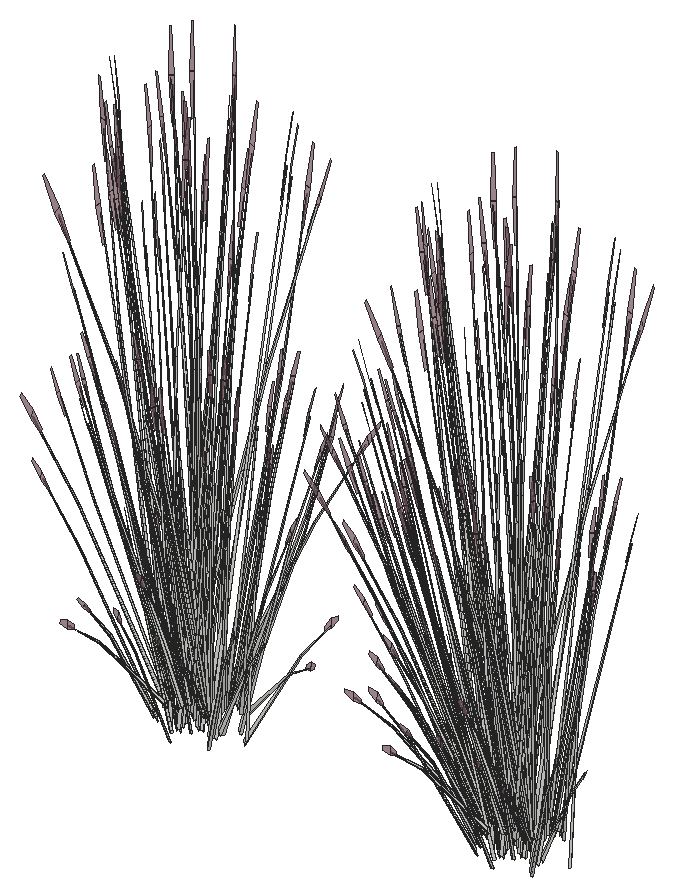
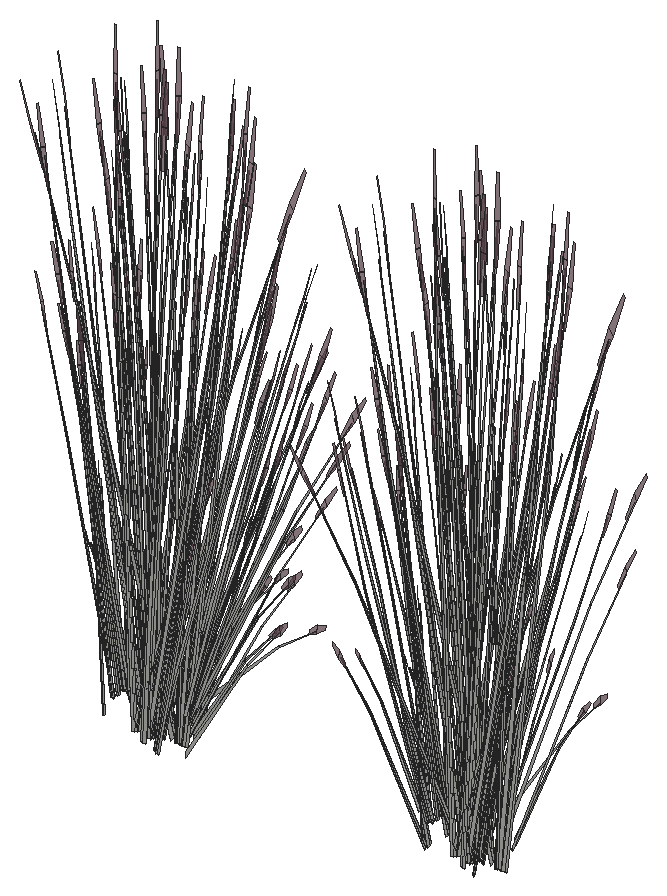
# SketchUp Ruby script. Lengths in inches.
U = 1.inch
M = Sketchup.active_model
def pt(a) = Geom::Point3d.new(a.map { |v| v * U })
def face(e, loops, mat)
  f = e.add_face(loops[0].map { |a| pt(a) })
  loops[1..].each { |l| e.add_face(l.map { |a| pt(a) }).erase! }
  f.material = f.back_material = mat if mat
  f
end
# faces: each face lists its corners as indices into pts; further lists are holes
def faces(e, pts, list, mat = nil) = list.each { |f| face(e, (f[0].is_a?(Array) ? f : [f]).map { |l| l.map { |i| pts[i] } }, mat) }
# xy, xz, yz: faces in a plane at the given z, y or x. An outline is a flat list of corners, or four numbers for a rectangle; further outlines are holes
def ring(l) = l.size == 4 ? [[l[0], l[1]], [l[2], l[1]], [l[2], l[3]], [l[0], l[3]]] : l.each_slice(2).to_a
def flat(e, list, mat, &to3) = list.each { |f| face(e, (f[0].is_a?(Array) ? f : [f]).map { |l| ring(l).map { |u, v| to3.(u, v) } }, mat) }
def xy(e, z, list, mat = nil) = flat(e, list, mat) { |x, y| [x, y, z] }
def xz(e, y, list, mat = nil) = flat(e, list, mat) { |x, z| [x, y, z] }
def yz(e, x, list, mat = nil) = flat(e, list, mat) { |y, z| [x, y, z] }
def lines(e, pts, list) = list.each { |a, b| e.add_line(pt(pts[a]), pt(pts[b])) }
# prism: a flat outline (further loops are holes) pulled along v
def prism(e, loops, v, mat = nil)
  f = face(e, loops, mat); d = Geom::Vector3d.new(v.map { |x| x * U })
  f.pushpull(f.normal.samedirection?(d) ? d.length : -d.length)
end
def box(e, o, s, mat = nil) = prism(e, [[o, [o[0] + s[0], o[1], o[2]], [o[0] + s[0], o[1] + s[1], o[2]], [o[0], o[1] + s[1], o[2]]]], [0, 0, s[2]], mat)
def at(x, y, z, deg = 0) = Geom::Transformation.translation(pt([x, y, z])) * Geom::Transformation.rotation(ORIGIN, Z_AXIS, deg.degrees)
def axes(o, x, y, z) = Geom::Transformation.new([*x, 0, *y, 0, *z, 0, *pt(o).to_a, 1])
def part(name) = M.definitions.add(name)
# library, detail: a bought-in or finely detailed component or shape, given as its bounding box
def library(name, o, s) = part(name).tap { |d| box(d.entities, o, s) }
def detail(e, o, s) = box(e.add_group.entities, o, s)
def put(e, d, t, mat = nil) = e.add_instance(d, t).tap { |i| i.material = mat if mat }
def group(e, t, mat = nil) = e.add_group.tap { |g| g.transformation = t; g.material = mat if mat }.entities
root = M.entities
M.materials.add("LightPink_Translucent").color = [144, 107, 117]
M.materials["LightPink_Translucent"].alpha = 0.75
c1 = part("blade")
p = [[2.15,0.21,22],[0,0.17,0],[0.09,0.45,0],[2.18,0.31,22],[2.29,0.31,22],[0.38,0.45,0],
  [2.48,0.24,33],[2.49,0.24,33],[2.48,0.22,33]]
faces(c1.entities,p,[[0,1,2,3],[4,5,2,3],[6,3,4,7],[8,0,3,6]])
c2 = part("seeds")
p = [[0.3,-0.1,1.38],[-0.01,-0.03,1.59],[-0.01,-0.03,0.03],[0.14,-0.07,-0.07],[0.29,-0.03,3],[0.15,0.01,3.11]]
faces(c2.entities,p,[[0,1,2,3],[1,0,4,5]],"LightPink_Translucent")
c3 = part("blade with seeds")
put(c3.entities,c1,at(0,0,0))
put(c3.entities,c2,axes([2.4,0.25,30.99],[1.5799,-0.05474,1.17369],[-0.12525,1.92788,0.29478],[-0.07173,-0.02425,1.56792]))
put(root,c3,axes([282.12,10.6,-2.125],[0.17368,0.19618,1.71376],[-0.80256,0.16516,0.13857],[-0.18139,-0.30799,0.73262]))
put(root,c3,axes([314.91,10.6,-2.125],[0.17368,0.19618,1.71376],[-0.80256,0.16516,0.13857],[-0.18139,-0.30799,0.73262]))
put(root,c3,axes([283.44,9.3,-1.28],[-0.11621,-0.08567,1.74944],[-0.77555,0.05431,-0.27667],[-0.12378,-0.20491,0.14031]))
put(root,c3,axes([316.24,9.3,-1.28],[-0.11621,-0.08567,1.74944],[-0.77555,0.05431,-0.27667],[-0.12378,-0.20491,0.14031]))
put(root,c3,axes([285.24,10.3125,-3.41],[-0.21597,0.12368,1.43002],[-0.64681,-0.21647,-0.30754],[0.1199,-0.26922,0.61141]))
put(root,c3,axes([318.03,10.3125,-3.41],[-0.21597,0.12368,1.43002],[-0.64681,-0.21647,-0.30754],[0.1199,-0.26922,0.61141]))
put(root,c3,axes([284.26,10.74,-1.02],[-0.36264,-0.49684,-0.71045],[0.74649,-0.27689,0.08574],[-0.0848,-0.24006,1.00501]))
put(root,c3,axes([317.05,10.74,-1.02],[-0.36264,-0.49684,-0.71045],[0.74649,-0.27689,0.08574],[-0.0848,-0.24006,1.00501]))
put(root,c3,axes([281.9,10.08,-3.41],[-0.04601,0.19989,1.43002],[-0.67263,0.16733,-0.30754],[-0.15723,-0.25836,0.61141]))
put(root,c3,axes([314.69,10.08,-3.41],[-0.04601,0.19989,1.43002],[-0.67263,0.16733,-0.30754],[-0.15723,-0.25836,0.61141]))
put(root,c3,axes([283.63,9.64,-4.51],[-0.12744,0.02202,1.76342],[-0.70477,-0.24781,-0.26939],[0.01183,-0.2067,0.30037]))
put(root,c3,axes([316.42,9.64,-4.51],[-0.12744,0.02202,1.76342],[-0.70477,-0.24781,-0.26939],[0.01183,-0.2067,0.30037]))
put(root,c3,axes([285.77,11.23,-1.02],[0.01977,-0.56521,-0.71045],[0.83252,0.03796,0.08574],[0.08786,-0.23945,1.00501]))
put(root,c3,axes([318.56,11.23,-1.02],[0.01977,-0.56521,-0.71045],[0.83252,0.03796,0.08574],[0.08786,-0.23945,1.00501]))
put(root,c3,axes([286.93,10.35,-1.28],[-0.00733,-0.12161,1.74944],[-0.61946,-0.35147,-0.27667],[0.09577,-0.21306,0.14031]))
put(root,c3,axes([319.72,10.35,-1.28],[-0.00733,-0.12161,1.74944],[-0.61946,-0.35147,-0.27667],[0.09577,-0.21306,0.14031]))
put(root,c3,axes([284.32,10.32,-1.47],[0.22906,-0.4699,-0.35414],[0.66828,0.13705,0.4572],[-0.06128,-0.18919,0.87481]))
put(root,c3,axes([317.12,10.32,-1.47],[0.22906,-0.4699,-0.35414],[0.66828,0.13705,0.4572],[-0.06128,-0.18919,0.87481]))
put(root,c3,axes([284.83,10.94,-2.125],[-0.14147,0.21002,1.71376],[-0.59349,-0.43464,0.13857],[0.26773,-0.27089,0.73262]))
put(root,c3,axes([317.62,10.94,-2.125],[-0.14147,0.21002,1.71376],[-0.59349,-0.43464,0.13857],[0.26773,-0.27089,0.73262]))
put(root,c3,axes([286.76,9.91,-1.29],[-0.07716,0.04667,1.77383],[-0.75601,-0.15746,-0.16761],[-0.02737,-0.20368,0.31391]))
put(root,c3,axes([319.55,9.91,-1.29],[-0.07716,0.04667,1.77383],[-0.75601,-0.15746,-0.16761],[-0.02737,-0.20368,0.31391]))
put(root,c3,axes([283.98,10.64,-1.32],[-0.7469,-0.15318,-0.51099],[0.25601,-0.52518,-0.3958],[-0.06849,-0.21144,0.97773]))
put(root,c3,axes([316.78,10.64,-1.32],[-0.7469,-0.15318,-0.51099],[0.25601,-0.52518,-0.3958],[-0.06849,-0.21144,0.97773]))
put(root,c3,axes([284.45,9.33,-3.23],[0.09747,0.35631,1.1486],[-0.54071,-0.19735,0.84392],[0.05818,-0.18244,0.25299]))
put(root,c3,axes([317.24,9.33,-3.23],[0.09747,0.35631,1.1486],[-0.54071,-0.19735,0.84392],[0.05818,-0.18244,0.25299]))
put(root,c3,axes([285.6,11.04,-1.32],[-0.54391,-0.41056,-0.51099],[0.57458,-0.35956,-0.3958],[0.08276,-0.2086,0.97773]))
put(root,c3,axes([318.39,11.04,-1.32],[-0.54391,-0.41056,-0.51099],[0.57458,-0.35956,-0.3958],[0.08276,-0.2086,0.97773]))
put(root,c3,axes([315.44,9.02,-1.29],[-0.01417,0.07324,1.77383],[-0.6991,0.2658,-0.16761],[-0.20573,-0.13587,0.31391]))
put(root,c3,axes([282.49,10.31,-0.91],[0.84639,-0.15705,0.53763],[0.14689,0.61608,0.4433],[-0.19906,-0.18157,1.11249]))
put(root,c3,axes([315.29,10.31,-0.91],[0.84639,-0.15705,0.53763],[0.14689,0.61608,0.4433],[-0.19906,-0.18157,1.11249]))
put(root,c3,axes([284.41,10.43,-1.27],[0.74868,0.15974,0.48003],[-0.25601,0.52518,0.3958],[-0.04499,-0.20653,0.9933]))
put(root,c3,axes([317.2,10.43,-1.27],[0.74868,0.15974,0.48003],[-0.25601,0.52518,0.3958],[-0.04499,-0.20653,0.9933]))
put(root,c3,axes([284.62,10.62,-0.97],[-0.74352,0.28449,-0.1216],[-0.36538,-0.50492,-0.67495],[-0.0981,-0.21277,1.02557]))
put(root,c3,axes([317.42,10.62,-0.97],[-0.74352,0.28449,-0.1216],[-0.36538,-0.50492,-0.67495],[-0.0981,-0.21277,1.02557]))
put(root,c3,axes([286.17,11.26,-0.97],[-0.83505,-0.03027,-0.1216],[0.02282,-0.57322,-0.67495],[0.05801,-0.22077,1.02557]))
put(root,c3,axes([318.96,11.26,-0.97],[-0.83505,-0.03027,-0.1216],[0.02282,-0.57322,-0.67495],[0.05801,-0.22077,1.02557]))
put(root,c3,axes([286.11,10.89,-1.47],[0.5141,-0.32171,-0.35414],[0.48666,0.36734,0.4572],[0.07405,-0.18664,0.87481]))
put(root,c3,axes([318.9,10.89,-1.47],[0.5141,-0.32171,-0.35414],[0.48666,0.36734,0.4572],[0.07405,-0.18664,0.87481]))
put(root,c3,axes([281.67,9.76,-3.23],[0.39634,0.21267,1.1486],[-0.57721,0.12784,0.84392],[-0.1235,-0.16344,0.25299]))
put(root,c3,axes([314.46,9.76,-3.23],[0.39634,0.21267,1.1486],[-0.57721,0.12784,0.84392],[-0.1235,-0.16344,0.25299]))
put(root,c3,axes([284.61,10.39,-1.27],[0.55987,-0.20767,0.0643],[0.27403,0.37869,0.50621],[-0.05407,-0.16693,0.77189]))
put(root,c3,axes([317.4,10.39,-1.27],[0.55987,-0.20767,0.0643],[0.27403,0.37869,0.50621],[-0.05407,-0.16693,0.77189]))
put(root,c3,axes([315.42,10.88,-1.02],[-0.64788,-0.29534,-0.71045],[0.46044,-0.51755,0.08574],[-0.23473,-0.17635,1.00501]))
put(root,c3,axes([282.4,10.49,-1.47],[-0.11735,-0.49217,-0.35414],[0.67083,-0.12996,0.4572],[-0.18018,-0.14104,0.87481]))
put(root,c3,axes([315.19,10.49,-1.47],[-0.11735,-0.49217,-0.35414],[0.67083,-0.12996,0.4572],[-0.18018,-0.14104,0.87481]))
put(root,c3,axes([282.6875,10.45,-1.27],[0.34533,-0.38816,0.0643],[0.49176,0.22599,0.50621],[-0.15898,-0.12445,0.77189]))
put(root,c3,axes([315.48,10.45,-1.27],[0.34533,-0.38816,0.0643],[0.49176,0.22599,0.50621],[-0.15898,-0.12445,0.77189]))
put(root,c3,axes([314.15,10.4,-4.51],[-0.0736,0.08049,1.76342],[-0.74378,0.17355,-0.26939],[-0.17968,-0.15788,0.30037]))
put(root,c3,axes([282.58,12.61,-3.9],[-0.31203,-0.62659,-0.69835],[0.89884,-0.22566,-0.18329],[-0.03449,-0.21218,1.54149]))
put(root,c3,axes([315.37,12.61,-3.9],[-0.31203,-0.62659,-0.69835],[0.89884,-0.22566,-0.18329],[-0.03449,-0.21218,1.54149]))
put(root,c3,axes([313.75,11.21,-2.125],[0.28223,0.10528,1.71376],[-0.58406,0.44165,0.13857],[-0.36402,-0.19924,0.73262]))
put(root,c3,axes([286.75,10.69,-4.51],[-0.11372,-0.04814,1.76342],[-0.29211,-0.53779,-0.26939],[0.19706,-0.14594,0.30037]))
put(root,c3,axes([319.54,10.69,-4.51],[-0.11372,-0.04814,1.76342],[-0.29211,-0.53779,-0.26939],[0.19706,-0.14594,0.30037]))
put(root,c3,axes([284.4,10.82,-0.95],[-0.22906,0.4699,0.35414],[-0.66828,-0.13705,-0.4572],[-0.06128,-0.18919,0.87481]))
put(root,c3,axes([317.19,10.82,-0.95],[-0.22906,0.4699,0.35414],[-0.66828,-0.13705,-0.4572],[-0.06128,-0.18919,0.87481]))
put(root,c3,axes([315.11,10.9,-1.32],[-0.74975,0.14525,-0.51099],[-0.13115,-0.55007,-0.3958],[-0.20138,-0.15763,0.97773]))
put(root,c3,axes([286.11,11.01,-1.27],[0.54105,0.41691,0.48003],[-0.57458,0.35956,0.3958],[0.0998,-0.1956,0.9933]))
put(root,c3,axes([318.9,11.01,-1.27],[0.54105,0.41691,0.48003],[-0.57458,0.35956,0.3958],[0.0998,-0.1956,0.9933]))
put(root,c3,axes([315.64,10.41,-0.57],[-0.50709,0.58578,-0.13619],[-0.73436,-0.33748,-0.75594],[-0.25527,-0.1655,1.14864]))
put(root,c3,axes([286.31,11.05,-1.27],[0.62439,0.02847,0.0643],[-0.01712,0.42991,0.50621],[0.06534,-0.16468,0.77189]))
put(root,c3,axes([319.1,11.05,-1.27],[0.62439,0.02847,0.0643],[-0.01712,0.42991,0.50621],[0.06534,-0.16468,0.77189]))
put(root,c3,axes([285.84,11.35,-0.95],[-0.5141,0.32171,0.35414],[-0.48666,-0.36734,-0.4572],[0.07405,-0.18664,0.87481]))
put(root,c3,axes([318.63,11.35,-0.95],[-0.5141,0.32171,0.35414],[-0.48666,-0.36734,-0.4572],[0.07405,-0.18664,0.87481]))
put(root,c3,axes([286.75,12.21,-1.02],[0.39688,-0.48213,-0.71045],[0.69548,0.34264,0.08574],[0.23697,-0.17468,1.00501]))
put(root,c3,axes([319.54,12.21,-1.02],[0.39688,-0.48213,-0.71045],[0.69548,0.34264,0.08574],[0.23697,-0.17468,1.00501]))
put(root,c3,axes([282.46,10.81,-3.625],[-0.47504,-0.61229,0],[0.79476,-0.34146,-0.51607],[0.18101,-0.07777,1.63711]))
put(root,c3,axes([315.25,10.81,-3.625],[-0.47504,-0.61229,0],[0.79476,-0.34146,-0.51607],[0.18101,-0.07777,1.63711]))
put(root,c3,axes([286.73,11.99,-1.32],[-0.19519,-0.55794,-0.51099],[0.73919,-0.0976,-0.3958],[0.21183,-0.14986,0.97773]))
put(root,c3,axes([319.52,11.99,-1.32],[-0.19519,-0.55794,-0.51099],[0.73919,-0.0976,-0.3958],[0.21183,-0.14986,0.97773]))
put(root,c3,axes([283.5,10.07,-3.87],[-0.52505,0.35054,-0.03893],[-0.48109,-0.38392,-0.17649],[-0.03387,-0.10878,0.58215]))
put(root,c3,axes([316.29,10.07,-3.87],[-0.52505,0.35054,-0.03893],[-0.48109,-0.38392,-0.17649],[-0.03387,-0.10878,0.58215]))
put(root,c3,axes([313.69,10.24,-1.28],[-0.16348,-0.00431,1.74944],[-0.52047,0.43131,-0.27667],[-0.2777,-0.08813,0.14031]))
put(root,c3,axes([287.08,12.39,-0.97],[-0.70283,-0.33692,-0.1216],[0.40491,-0.48793,-0.67495],[0.19857,-0.16961,1.02557]))
put(root,c3,axes([319.87,12.39,-0.97],[-0.70283,-0.33692,-0.1216],[0.40491,-0.48793,-0.67495],[0.19857,-0.16961,1.02557]))
put(root,c3,axes([284.17,14.22,-2.67],[0.65659,0.2464,1.51261],[-0.64324,0.53082,0.59816],[-0.28812,-0.31461,1.26806]))
put(root,c3,axes([316.97,14.22,-2.67],[0.65659,0.2464,1.51261],[-0.64324,0.53082,0.59816],[-0.28812,-0.31461,1.26806]))
put(root,c3,axes([282.79,10.89,-0.95],[0.11735,0.49217,0.35414],[-0.67083,0.12996,-0.4572],[-0.18018,-0.14104,0.87481]))
put(root,c3,axes([315.59,10.89,-0.95],[0.11735,0.49217,0.35414],[-0.67083,0.12996,-0.4572],[-0.18018,-0.14104,0.87481]))
put(root,c3,axes([280.74,12.52,-3.98],[0,-0.61104,-0.49651],[0.85008,0,0],[0,-0.13917,1.57504]))
put(root,c3,axes([313.53,12.52,-3.98],[0,-0.61104,-0.49651],[0.85008,0,0],[0,-0.13917,1.57504]))
put(root,c3,axes([283.1,10.71,-3.98],[0.7111,-0.30552,-0.49651],[0.42504,0.54784,0],[0.16196,-0.06958,1.57504]))
put(root,c3,axes([315.9,10.71,-3.98],[0.7111,-0.30552,-0.49651],[0.42504,0.54784,0],[0.16196,-0.06958,1.57504]))
put(root,c3,axes([287.32,11.77,-3.41],[-0.27143,-0.0181,1.43002],[-0.27808,-0.48551,-0.30754],[0.33346,-0.13735,0.61141]))
put(root,c3,axes([313.57,11.21,-0.91],[0.62747,-0.45094,0.53763],[0.54116,0.47889,0.4433],[-0.29439,-0.08318,1.11249]))
put(root,c3,axes([288.81,12.24,-1.29],[-0.09924,-0.00464,1.77383],[-0.4121,-0.49725,-0.16761],[0.1655,-0.1635,0.31391]))
put(root,c3,axes([321.6,12.24,-1.29],[-0.09924,-0.00464,1.77383],[-0.4121,-0.49725,-0.16761],[0.1655,-0.1635,0.31391]))
put(root,c3,axes([283.94,11.97,-3.94],[0.51177,-0.45928,-0.62353],[0.63575,0.41646,-0.16365],[0.20507,-0.11457,1.37633]))
put(root,c3,axes([316.74,11.97,-3.94],[0.51177,-0.45928,-0.62353],[0.63575,0.41646,-0.16365],[0.20507,-0.11457,1.37633]))
put(root,c3,axes([287.63,10.875,-3.23],[-0.25308,0.31105,1.1486],[-0.21753,-0.4179,0.84392],[0.20902,-0.10472,0.25299]))
put(root,c3,axes([320.43,10.875,-3.23],[-0.25308,0.31105,1.1486],[-0.21753,-0.4179,0.84392],[0.20902,-0.10472,0.25299]))
put(root,c3,axes([287.27,12.04,-1.47],[0.66138,-0.08733,-0.35414],[0.17464,0.49921,0.4572],[0.18953,-0.13408,0.87481]))
put(root,c3,axes([320.07,12.04,-1.47],[0.66138,-0.08733,-0.35414],[0.17464,0.49921,0.4572],[0.18953,-0.13408,0.87481]))
put(root,c3,axes([313.86,11.21,-1.27],[0.03826,-0.46465,0.0643],[0.57772,0.01274,0.50621],[-0.2213,-0.04862,0.77189]))
put(root,c3,axes([283.05,12.77,-3.79],[0.36864,-0.55059,-0.44739],[0.76598,0.26498,0.21531],[0,-0.12692,1.43643]))
put(root,c3,axes([315.85,12.77,-3.79],[0.36864,-0.55059,-0.44739],[0.76598,0.26498,0.21531],[0,-0.12692,1.43643]))
put(root,c3,axes([313.64,11.36,-1.47],[-0.43232,-0.38257,-0.35414],[0.49364,-0.36215,0.4572],[-0.25081,-0.0551,0.87481]))
put(root,c3,axes([283.39,12.5,-3.33],[-0.08854,-0.69723,-0.29095],[0.92215,-0.04216,-0.50002],[0.16238,-0.09287,1.59708]))
put(root,c3,axes([316.18,12.5,-3.33],[-0.08854,-0.69723,-0.29095],[0.92215,-0.04216,-0.50002],[0.16238,-0.09287,1.59708]))
put(root,c3,axes([281.1,12.54,-3.97],[0.53038,-0.38124,-0.30978],[0.53038,0.38124,0.30978],[0,-0.1228,1.38974]))
put(root,c3,axes([313.9,12.54,-3.97],[0.53038,-0.38124,-0.30978],[0.53038,0.38124,0.30978],[0,-0.1228,1.38974]))
put(root,c3,axes([313.68,10.71,-3.87],[-0.21918,0.49894,-0.03893],[-0.6746,-0.15348,-0.17649],[-0.10242,-0.08161,0.58215]))
put(root,c3,axes([286.73,12.34,-0.95],[-0.66138,0.08733,0.35414],[-0.17464,-0.49921,-0.4572],[0.18953,-0.13408,0.87481]))
put(root,c3,axes([319.53,12.34,-0.95],[-0.66138,0.08733,0.35414],[-0.17464,-0.49921,-0.4572],[0.18953,-0.13408,0.87481]))
put(root,c3,axes([282.96,13.23,-3.33],[-0.85568,-0.29155,-0.29095],[0.41201,-0.61537,-0.50002],[-0.02689,-0.15109,1.59708]))
put(root,c3,axes([315.76,13.23,-3.33],[-0.85568,-0.29155,-0.29095],[0.41201,-0.61537,-0.50002],[-0.02689,-0.15109,1.59708]))
put(root,c3,axes([280.53,12.99,-3.625],[-0.95008,0,0],[0,-0.68292,-0.51607],[0,-0.15554,1.63711]))
put(root,c3,axes([313.32,12.99,-3.625],[-0.95008,0,0],[0,-0.68292,-0.51607],[0,-0.15554,1.63711]))
put(root,c3,axes([313.48,11.76,-3.41],[0.14835,0.17012,1.43002],[-0.34183,0.46242,-0.30754],[-0.351,-0.11053,0.61141]))
put(root,c3,axes([283.27,10.95,-3.97],[0.70886,0.15119,-0.30978],[-0.17848,0.53243,0.30978],[0.1429,-0.0614,1.38974]))
put(root,c3,axes([316.0625,10.95,-3.97],[0.70886,0.15119,-0.30978],[-0.17848,0.53243,0.30978],[0.1429,-0.0614,1.38974]))
put(root,c3,axes([314.1,11.61,-1.02],[-0.75952,-0.01471,-0.71045],[0.05101,-0.61953,0.08574],[-0.32177,-0.06538,1.00501]))
put(root,c3,axes([287.33,12.26,-1.27],[0.52161,0.25698,0.0643],[-0.30368,0.36595,0.50621],[0.16723,-0.11831,0.77189]))
put(root,c3,axes([320.125,12.26,-1.27],[0.52161,0.25698,0.0643],[-0.30368,0.36595,0.50621],[0.16723,-0.11831,0.77189]))
put(root,c3,axes([287.1875,12.15,-1.27],[0.18844,0.56237,0.48003],[-0.73919,0.0976,0.3958],[0.21785,-0.13226,0.9933]))
put(root,c3,axes([319.98,12.15,-1.27],[0.18844,0.56237,0.48003],[-0.73919,0.0976,0.3958],[0.21785,-0.13226,0.9933]))
put(root,c3,axes([289.18,12.83,-1.28],[0.10543,-0.09307,1.74944],[-0.13495,-0.57092,-0.27667],[0.26455,-0.10825,0.14031]))
put(root,c3,axes([281.26,12.81,-3.67],[-0.70674,0.51372,0.30756],[-0.70717,-0.50832,-0.36492],[-0.02468,-0.14589,1.64885]))
put(root,c3,axes([314.06,12.81,-3.67],[-0.70674,0.51372,0.30756],[-0.70717,-0.50832,-0.36492],[-0.02468,-0.14589,1.64885]))
put(root,c3,axes([313.0625,10.6,-1.29],[0.05633,0.06098,1.77383],[-0.27155,0.54815,-0.16761],[-0.27501,0.00397,0.31391]))
put(root,c3,axes([283.51,13.04,-3.57],[0.8561,0.29616,0.24065],[-0.41201,0.61537,0.50002],[0,-0.14185,1.60543]))
put(root,c3,axes([316.3,13.04,-3.57],[0.8561,0.29616,0.24065],[-0.41201,0.61537,0.50002],[0,-0.14185,1.60543]))
put(root,c3,axes([283.18,13.875,-3.5625],[0.20138,-0.72405,-0.23429],[0.95485,0.12621,0.51271],[-0.16685,-0.09999,1.5644]))
put(root,c3,axes([315.97,13.875,-3.5625],[0.20138,-0.72405,-0.23429],[0.95485,0.12621,0.51271],[-0.16685,-0.09999,1.5644]))
put(root,c3,axes([313.84,11.74,-1.32],[-0.55171,0.40476,-0.51099],[-0.48318,-0.42758,-0.3958],[-0.28031,-0.06159,0.97773]))
put(root,c3,axes([314.25,11.56,-0.95],[0.43232,0.38257,0.35414],[-0.49364,0.36215,-0.4572],[-0.25081,-0.0551,0.87481]))
put(root,c3,axes([312.6,12.28,-3.23],[0.48508,-0.04372,1.1486],[-0.3077,0.38525,0.84392],[-0.23971,-0.05779,0.25299]))
put(root,c3,axes([283.23,12.63,-3.28],[-0.82508,0.03772,0.44739],[-0.07462,-0.62614,-0.21531],[0.14771,-0.06346,1.43643]))
put(root,c3,axes([316.03,12.63,-3.28],[-0.82508,0.03772,0.44739],[-0.07462,-0.62614,-0.21531],[0.14771,-0.06346,1.43643]))
put(root,c3,axes([314.13,11.32,-0.97],[-0.04068,0.62141,-0.1216],[-0.77029,-0.01698,-0.67495],[-0.29667,-0.04317,1.02557]))
put(root,c3,axes([281.1,13.09,-3.52],[0,0.61104,0.49651],[-0.85008,0,0],[0,-0.13917,1.57504]))
put(root,c3,axes([313.9,13.09,-3.52],[0,0.61104,0.49651],[-0.85008,0,0],[0,-0.13917,1.57504]))
put(root,c3,axes([287.1,13.7,-0.97],[-0.38229,-0.5533,-0.1216],[0.6785,-0.2719,-0.67495],[0.28593,-0.073,1.02557]))
put(root,c3,axes([319.9,13.7,-0.97],[-0.38229,-0.5533,-0.1216],[0.6785,-0.2719,-0.67495],[0.28593,-0.073,1.02557]))
put(root,c3,axes([287.07,13.22,-1.32],[0.20584,-0.55581,-0.51099],[0.70573,0.19051,-0.3958],[0.28414,-0.05097,0.97773]))
put(root,c3,axes([319.86,13.22,-1.32],[0.20584,-0.55581,-0.51099],[0.70573,0.19051,-0.3958],[0.28414,-0.05097,0.97773]))
put(root,c3,axes([285.95,10.96,-3.625],[0.47504,-0.61229,0],[0.79476,0.34146,-0.51607],[0.18101,0.07777,1.63711]))
put(root,c3,axes([318.75,10.96,-3.625],[0.47504,-0.61229,0],[0.79476,0.34146,-0.51607],[0.18101,0.07777,1.63711]))
put(root,c3,axes([313.15,12.17,-2.125],[0.31515,-0.01384,1.71376],[-0.20907,0.5998,0.13857],[-0.44912,-0.0371,0.73262]))
put(root,c3,axes([283.11,13.58,-3.79],[-0.45644,-0.51287,-0.44739],[0.69137,-0.36116,0.21531],[-0.14771,-0.06346,1.43643]))
put(root,c3,axes([315.9,13.58,-3.79],[-0.45644,-0.51287,-0.44739],[0.69137,-0.36116,0.21531],[-0.14771,-0.06346,1.43643]))
put(root,c3,axes([283.21,12.86,-3.64],[0.33034,0.68327,0.45755],[-0.94388,0.2376,0.17955],[0.01154,-0.12555,1.58856]))
put(root,c3,axes([316,12.86,-3.64],[0.33034,0.68327,0.45755],[-0.94388,0.2376,0.17955],[0.01154,-0.12555,1.58856]))
put(root,c3,axes([287.82,13.38,-4.02],[-0.48937,0.07333,1.41583],[-0.07789,-0.58369,0.08104],[0.34275,-0.08835,0.80566]))
put(root,c3,axes([288.72,12.86,-3.74],[-0.47106,-0.39072,-0.06488],[0.51591,-0.35801,-0.29416],[0.14618,-0.02521,0.97024]))
put(root,c3,axes([321.51,12.86,-3.74],[-0.47106,-0.39072,-0.06488],[0.51591,-0.35801,-0.29416],[0.14618,-0.02521,0.97024]))
put(root,c3,axes([283.04,13.4,-3.28],[-0.36864,0.55059,0.44739],[-0.76598,-0.26498,-0.21531],[0,-0.12692,1.43643]))
put(root,c3,axes([315.83,13.4,-3.28],[-0.36864,0.55059,0.44739],[-0.76598,-0.26498,-0.21531],[0,-0.12692,1.43643]))
put(root,c3,axes([284.39,12.92,-3.79],[0,-0.70701,0],[0.95008,0,0],[0,0,1.79456]))
put(root,c3,axes([317.1875,12.92,-3.79],[0,-0.70701,0],[0.95008,0,0],[0,0,1.79456]))
put(root,c3,axes([285.55,11.28,-3.52],[-0.7111,-0.30552,0.49651],[0.42504,-0.54784,0],[0.16196,0.06958,1.57504]))
put(root,c3,axes([318.34,11.28,-3.52],[-0.7111,-0.30552,0.49651],[0.42504,-0.54784,0],[0.16196,0.06958,1.57504]))
put(root,c3,axes([286.9375,13.43,-1.02],[0.66765,-0.26986,-0.71045],[0.37208,0.55551,0.08574],[0.32259,-0.0631,1.00501]))
put(root,c3,axes([315.49,13.78,-3.94],[-0.79037,-0.10018,-0.62353],[0.16679,-0.61794,-0.16365],[-0.23587,-0.07488,1.37633]))
put(root,c3,axes([283.94,12.47,-3.64],[-0.62999,0.55453,0.45755],[-0.74845,-0.4895,0.17955],[0.15188,-0.05534,1.58856]))
put(root,c3,axes([316.74,12.47,-3.64],[-0.62999,0.55453,0.45755],[-0.74845,-0.4895,0.17955],[0.15188,-0.05534,1.58856]))
put(root,c3,axes([284.63,13.46,-3.7],[-0.70674,-0.52593,-0.06131],[0.70717,-0.52625,0],[-0.02468,-0.01837,1.75571]))
put(root,c3,axes([317.42,13.46,-3.7],[-0.70674,-0.52593,-0.06131],[0.70717,-0.52625,0],[-0.02468,-0.01837,1.75571]))
put(root,c3,axes([282.85,11.56,-3.53],[-0.21949,0.60727,0.17642],[-0.8032,-0.17185,0.35086],[0.13875,-0.00296,1.60407]))
put(root,c3,axes([315.64,11.56,-3.53],[-0.21949,0.60727,0.17642],[-0.8032,-0.17185,0.35086],[0.13875,-0.00296,1.60407]))
put(root,c3,axes([286.84,13.53,-0.95],[-0.63144,-0.17046,0.35414],[0.18417,-0.49731,-0.4572],[0.25423,-0.0456,0.87481]))
put(root,c3,axes([319.63,13.53,-0.95],[-0.63144,-0.17046,0.35414],[0.18417,-0.49731,-0.4572],[0.25423,-0.0456,0.87481]))
put(root,c3,axes([313.02,12.625,-1.27],[0.21466,-0.55714,0.48003],[0.70573,0.19051,0.3958],[-0.27753,0.03348,0.9933]))
put(root,c3,axes([282.52,12.05,-4.41],[-0.74787,0.24464,1.28929],[-0.23804,-0.70192,0.50096],[0.45924,0.01168,1.46642]))
put(root,c3,axes([315.3125,12.05,-4.41],[-0.74787,0.24464,1.28929],[-0.23804,-0.70192,0.50096],[0.45924,0.01168,1.46642]))
put(root,c3,axes([284.53,12.23,-3.38],[0.14658,-0.54532,0.1448],[0.71613,0.09466,-0.41347],[0.13033,0.05599,1.26744]))
put(root,c3,axes([317.32,12.23,-3.38],[0.14658,-0.54532,0.1448],[0.71613,0.09466,-0.41347],[0.13033,0.05599,1.26744]))
put(root,c3,axes([312.97,12.48,-1.27],[-0.27906,-0.41663,0.0643],[0.50888,-0.20393,0.50621],[-0.22432,0.04024,0.77189]))
put(root,c3,axes([283.29,13.53,-3.64],[0.96033,0.12874,0.45755],[-0.19544,0.7271,0.17955],[-0.14034,-0.07021,1.58856]))
put(root,c3,axes([316.08,13.53,-3.64],[0.96033,0.12874,0.45755],[-0.19544,0.7271,0.17955],[-0.14034,-0.07021,1.58856]))
put(root,c3,axes([288.36,13,-4.51],[-0.03971,-0.09277,1.76342],[0.27541,-0.54264,-0.26939],[0.27782,-0.00781,0.30037]))
put(root,c3,axes([312.95,12.91,-4.51],[0.01927,0.0963,1.76342],[-0.38846,0.5029,-0.26939],[-0.27592,-0.02535,0.30037]))
put(root,c3,axes([284.22,12.375,-3.28],[-0.45644,-0.51287,0.44739],[0.69137,-0.36116,-0.21531],[0.14771,0.06346,1.43643]))
put(root,c3,axes([317.01,12.375,-3.28],[-0.45644,-0.51287,0.44739],[0.69137,-0.36116,-0.21531],[0.14771,0.06346,1.43643]))
put(root,c3,axes([281.86,14.72,-3.97],[-0.17848,-0.53243,-0.30978],[0.70886,-0.15119,0.30978],[-0.1429,-0.0614,1.38974]))
put(root,c3,axes([314.66,14.72,-3.97],[-0.17848,-0.53243,-0.30978],[0.70886,-0.15119,0.30978],[-0.1429,-0.0614,1.38974]))
put(root,c3,axes([282.77,14.6875,-3.53],[0.81646,-0.16218,0.17642],[0.20161,0.60355,0.35086],[-0.07282,-0.08794,1.60407]))
put(root,c3,axes([315.57,14.6875,-3.53],[0.81646,-0.16218,0.17642],[0.20161,0.60355,0.35086],[-0.07282,-0.08794,1.60407]))
put(root,c3,axes([284.45,12.41,-3.33],[0.76714,-0.40567,-0.29095],[0.51013,0.57321,-0.50002],[0.18927,0.05821,1.59708]))
put(root,c3,axes([317.25,12.41,-3.33],[0.76714,-0.40567,-0.29095],[0.51013,0.57321,-0.50002],[0.18927,0.05821,1.59708]))
put(root,c3,axes([287.5,13.48,-1.47],[0.63144,0.17046,-0.35414],[-0.18417,0.49731,0.4572],[0.25423,-0.0456,0.87481]))
put(root,c3,axes([314.46,14.95,-3.98],[-0.7111,-0.30552,-0.49651],[0.42504,-0.54784,0],[-0.16196,-0.06958,1.57504]))
put(root,c3,axes([286.39,11.33,-3.98],[0.7111,0.30552,-0.49651],[-0.42504,0.54784,0],[0.16196,0.06958,1.57504]))
put(root,c3,axes([319.18,11.33,-3.98],[0.7111,0.30552,-0.49651],[-0.42504,0.54784,0],[0.16196,0.06958,1.57504]))
put(root,c3,axes([312.875,12.6875,-1.47],[-0.63144,-0.17046,-0.35414],[0.18417,-0.49731,0.4572],[-0.25423,0.0456,0.87481]))
put(root,c3,axes([285.04,13.07,-3.79],[0.85008,0,0],[0,0.63259,0],[0,0,1.78407]))
put(root,c3,axes([317.83,13.07,-3.79],[0.85008,0,0],[0,0.63259,0],[0,0,1.78407]))
put(root,c3,axes([283.6,13.87,-3.33],[-0.76714,0.40567,-0.29095],[-0.51013,-0.57321,-0.50002],[-0.18927,-0.05821,1.59708]))
put(root,c3,axes([316.39,13.87,-3.33],[-0.76714,0.40567,-0.29095],[-0.51013,-0.57321,-0.50002],[-0.18927,-0.05821,1.59708]))
put(root,c3,axes([285.28,11.59,-3.53],[-0.81646,0.16218,0.17642],[-0.20161,-0.60355,0.35086],[0.07282,0.08794,1.60407]))
put(root,c3,axes([318.07,11.59,-3.53],[-0.81646,0.16218,0.17642],[-0.20161,-0.60355,0.35086],[0.07282,0.08794,1.60407]))
put(root,c3,axes([285.78,12.86,-2.125],[-0.31515,0.01384,1.71376],[0.20907,-0.5998,0.13857],[0.44912,0.0371,0.73262]))
